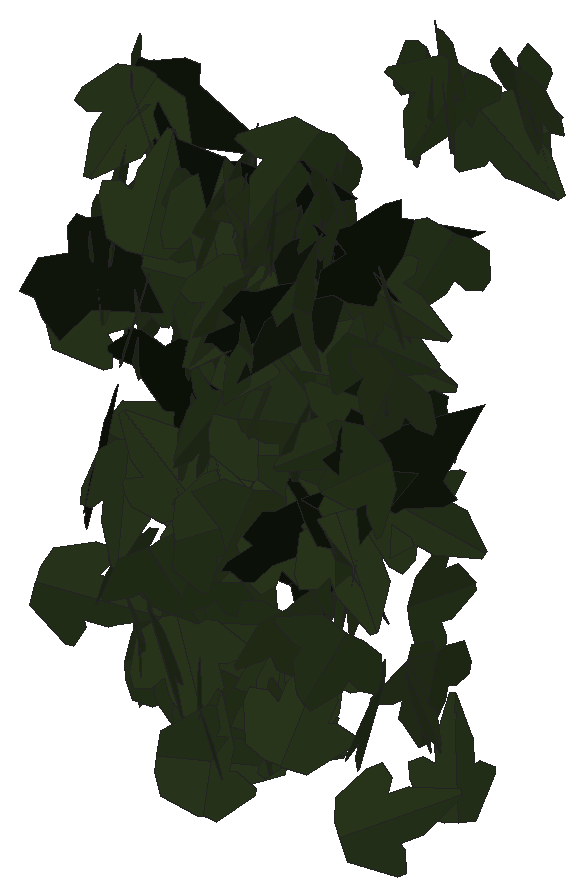
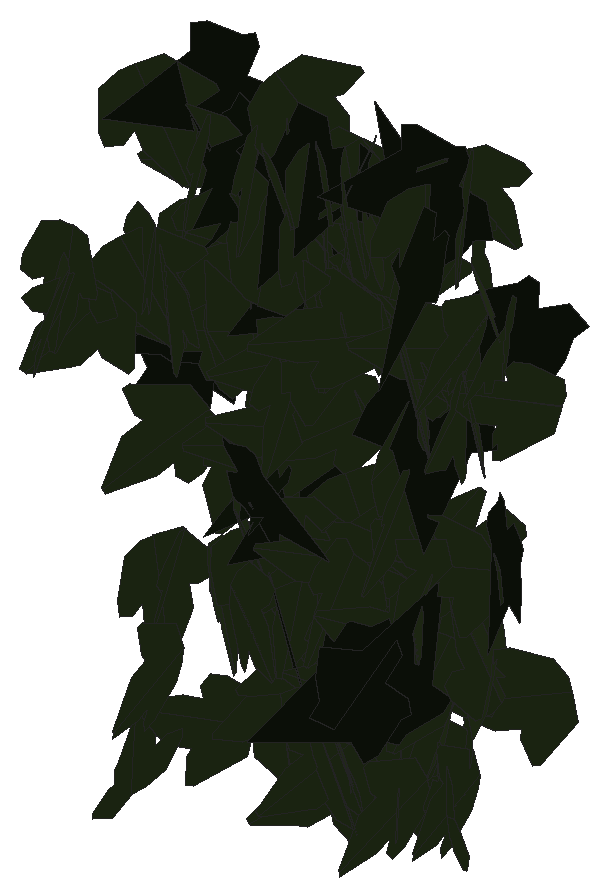
# SketchUp Ruby script. Lengths in inches.
U = 1.inch
M = Sketchup.active_model
def pt(a) = Geom::Point3d.new(a.map { |v| v * U })
def face(e, loops, mat)
  f = e.add_face(loops[0].map { |a| pt(a) })
  loops[1..].each { |l| e.add_face(l.map { |a| pt(a) }).erase! }
  f.material = f.back_material = mat if mat
  f
end
# faces: each face lists its corners as indices into pts; further lists are holes
def faces(e, pts, list, mat = nil) = list.each { |f| face(e, (f[0].is_a?(Array) ? f : [f]).map { |l| l.map { |i| pts[i] } }, mat) }
# xy, xz, yz: faces in a plane at the given z, y or x. An outline is a flat list of corners, or four numbers for a rectangle; further outlines are holes
def ring(l) = l.size == 4 ? [[l[0], l[1]], [l[2], l[1]], [l[2], l[3]], [l[0], l[3]]] : l.each_slice(2).to_a
def flat(e, list, mat, &to3) = list.each { |f| face(e, (f[0].is_a?(Array) ? f : [f]).map { |l| ring(l).map { |u, v| to3.(u, v) } }, mat) }
def xy(e, z, list, mat = nil) = flat(e, list, mat) { |x, y| [x, y, z] }
def xz(e, y, list, mat = nil) = flat(e, list, mat) { |x, z| [x, y, z] }
def yz(e, x, list, mat = nil) = flat(e, list, mat) { |y, z| [x, y, z] }
def lines(e, pts, list) = list.each { |a, b| e.add_line(pt(pts[a]), pt(pts[b])) }
# prism: a flat outline (further loops are holes) pulled along v
def prism(e, loops, v, mat = nil)
  f = face(e, loops, mat); d = Geom::Vector3d.new(v.map { |x| x * U })
  f.pushpull(f.normal.samedirection?(d) ? d.length : -d.length)
end
def box(e, o, s, mat = nil) = prism(e, [[o, [o[0] + s[0], o[1], o[2]], [o[0] + s[0], o[1] + s[1], o[2]], [o[0], o[1] + s[1], o[2]]]], [0, 0, s[2]], mat)
def at(x, y, z, deg = 0) = Geom::Transformation.translation(pt([x, y, z])) * Geom::Transformation.rotation(ORIGIN, Z_AXIS, deg.degrees)
def axes(o, x, y, z) = Geom::Transformation.new([*x, 0, *y, 0, *z, 0, *pt(o).to_a, 1])
def part(name) = M.definitions.add(name)
# library, detail: a bought-in or finely detailed component or shape, given as its bounding box
def library(name, o, s) = part(name).tap { |d| box(d.entities, o, s) }
def detail(e, o, s) = box(e.add_group.entities, o, s)
def put(e, d, t, mat = nil) = e.add_instance(d, t).tap { |i| i.material = mat if mat }
def group(e, t, mat = nil) = e.add_group.tap { |g| g.transformation = t; g.material = mat if mat }.entities
root = M.entities
M.materials.add("efeu1").color = [18, 25, 13]
M.materials.add("efeu2").color = [43, 57, 29]
c1 = part("ivyleaf_9")
p = [[1.54,2.16,1.25],[1.36,2.04,1.19],[-0.21,0.99,0.68],[-0.71,1.11,0.82],[-0.85,0.86,0.67],[-0.8,0.17,0.21],
  [-0.9,-0.01,0.1],[-0.67,-0.16,-0.02],[-0.08,-0.08,-0.05],[-0.03,-0.6,-0.4],[0.65,-0.88,-0.66],[0.83,-0.6,-0.49],
  [1.29,-0.42,-0.43],[1.8125,-0.07,-0.26],[1.21,0.44,0.15]]
faces(c1.entities,p,[[0,1,2,3,4,5,6,7,8,9,10,11,12,13,14]],"efeu1")
c2 = part("ivyleaf_10")
p = [[0,0.5,-0.03],[-0.0625,2.02,-0.43],[-0.19,2.01,-0.46],[-0.54,1.05,-0.29],[-0.52,0.625,-0.18],[-0.83,0.76,-0.28],
  [-1.16,0.64,-0.33],[-1.15,0.33,-0.24],[-0.77,-0.39,0.02],[-0.3,-0.51,0.16],[0.04,-0.48,0.23],[-0.02,2.01,-0.4375],
  [-0.06,2.01,-0.43],[0.04,-0.49,0.23],[0.67,-0.49,0.14],[1.38,0.36,-0.2],[1.375,0.51,-0.24],[0.81,0.65,-0.19],
  [0.62,0.59,-0.15],[0.6,1.09,-0.28],[0.5,1.23,-0.31]]
faces(c2.entities,p,[[0,1,2,3,4,5,6,7,8,9,10],[11,12,0,13,14,15,16,17,18,19,20]],"efeu2")
put(root,c1,axes([22.51,224.58,212.38],[0.06271,-0.08409,-0.48887],[-0.01576,0.49218,-0.08668],[0.4958,0.02628,0.05908]))
put(root,c2,axes([23.38,224.66,212.97],[0.22592,0.39135,-0.21402],[0.09036,0.19477,0.45155],[0.4368,-0.24271,0.01728]))
put(root,c2,axes([26.13,224.89,208.42],[0.18941,-0.45118,-0.10279],[-0.04536,0.09243,-0.48929],[0.46051,0.19467,-0.00592]))
put(root,c2,axes([24.34,225.04,212.48],[0.30249,0.28815,-0.27471],[-0.21033,-0.17727,-0.41754],[-0.33802,0.36817,0.01397]))
put(root,c2,axes([25.64,224.95,208.82],[-0.40532,-0.15765,0.24671],[-0.22122,-0.11108,-0.43442],[0.19178,-0.46131,0.02029]))
put(root,c2,axes([26.13,224.84,211.12],[0.30736,-0.11212,-0.3781],[-0.33453,0.17974,-0.32524],[0.20885,0.4529,0.03547]))
put(root,c2,axes([25.46,224.61,212.77],[-0.1703,0.22314,0.41377],[-0.25775,0.32372,-0.28067],[-0.39314,-0.30889,0.00477]))
put(root,c2,axes([26.38,224.9,212.14],[-0.43486,-0.04069,0.24339],[-0.24112,-0.03479,-0.43663],[0.05247,-0.49713,0.01064]))
put(root,c2,axes([25.77,225.1,211.27],[-0.2106,-0.12766,0.43514],[-0.34341,-0.26845,-0.24496],[0.29618,-0.40204,0.02539]))
put(root,c2,axes([22.2,224.8,208.38],[-0.12391,-0.03449,-0.48317],[0.47025,0.11113,-0.12853],[0.11625,-0.48627,0.0049]))
put(root,c1,axes([26.12,224.55,213.6875],[0.03425,0.24336,-0.43544],[-0.01395,0.43676,0.243],[0.49863,-0.00449,0.0367]))
put(root,c2,axes([24.27,225.04,212.37],[0.07229,-0.49389,0.02911],[0.00313,-0.02896,-0.49915],[0.49474,0.07235,-0.0011]))
put(root,c2,axes([22.88,225,209.91],[0.18698,0.45081,-0.10866],[-0.03926,-0.10135,-0.48804],[-0.46206,0.19104,-0.0025]))
put(root,c2,axes([24.51,224.74,211.96],[0.038,-0.05493,-0.49552],[-0.35423,0.34672,-0.0656],[0.35082,0.35604,-0.01257]))
put(root,c2,axes([25.12,224.77,207.64],[0.29397,0.32785,-0.23685],[0.16042,0.17427,0.44034],[0.37128,-0.33488,-0.00272]))
put(root,c1,axes([25.3,225.11,212.84],[-0.48907,0.07078,-0.07613],[0.07511,-0.01256,-0.49417],[-0.07186,-0.49481,0.00165]))
put(root,c2,axes([23.9375,225.2,213.18],[0.17877,-0.41132,0.22104],[0.10171,-0.1967,-0.44829],[0.45574,0.20524,0.01334]))
put(root,c2,axes([25.97,224.99,213.1],[-0.18972,-0.01175,-0.46246],[0.45973,-0.0605,-0.18706],[-0.05156,-0.49619,0.03376]))
put(root,c2,axes([23.85,224.96,206.61],[0.4903,-0.09038,-0.03797],[0.03745,-0.00629,0.49856],[-0.0906,-0.49172,0.0006]))
put(root,c2,axes([22.71,225.24,208.08],[-0.15403,-0.02039,0.47525],[0.41493,-0.25004,0.12375],[0.23262,0.43251,0.09395]))
put(root,c2,axes([23.98,224.66,209.67],[0.0492,-0.0791,-0.49125],[0.22622,0.44323,-0.04871],[0.44318,-0.21747,0.0794]))
put(root,c2,axes([24.125,224.95,211.59],[0.48591,-0.08464,-0.08204],[0.0858,0.01531,0.49235],[-0.08083,-0.49255,0.02941]))
put(root,c2,axes([24.32,225.1,209.92],[-0.33701,-0.32758,0.17064],[-0.11137,-0.13013,-0.46975],[0.35217,-0.35463,0.01475]))
put(root,c2,axes([24.98,225.23,214.2],[-0.23374,-0.33714,0.28584],[-0.10346,-0.27263,-0.40617],[0.42973,-0.24901,0.05769]))
put(root,c1,axes([23.33,225.2,213.2],[-0.05496,0.02126,0.49651],[0.27897,-0.41209,0.04852],[0.41128,0.28236,0.03344]))
put(root,c2,axes([23.92,224.99,213.36],[0.25014,0.43015,0.04902],[0.02474,0.04232,-0.49759],[-0.43222,0.25136,-0.00011]))
put(root,c2,axes([25.02,225.03,211.14],[-0.13159,0.03096,0.48138],[-0.47888,-0.06829,-0.12652],[0.05791,-0.49435,0.04763]))
put(root,c2,axes([23.77,224.77,206.93],[0.03196,0.02339,0.49843],[0.29196,0.40415,-0.03769],[-0.40464,0.29346,0.01217]))
put(root,c2,axes([22.29,224.82,211.55],[0.13795,-0.00364,-0.48058],[0.41394,0.25493,0.11689],[0.24417,-0.43012,0.07335]))
put(root,c2,axes([23.71,225.1875,212.69],[-0.43376,-0.21923,-0.11744],[-0.09322,-0.07558,0.48538],[-0.23057,0.44298,0.0247]))
put(root,c2,axes([23.63,225.42,210.61],[-0.0463,-0.01692,0.49756],[0.24111,-0.43796,0.00755],[0.43557,0.24063,0.04872]))
put(root,c1,axes([24.55,224.72,212.27],[0.31579,0.25777,0.28954],[0.22934,0.17686,-0.40759],[-0.31254,0.39023,-0.00653]))
put(root,c2,axes([22.5625,225.3125,213.11],[0.25774,-0.26249,0.33862],[0.24668,-0.23218,-0.36775],[0.35031,0.35664,0.00982]))
put(root,c2,axes([23.3125,224.94,209.01],[-0.31521,-0.32538,-0.21159],[0.13739,0.16139,-0.45286],[0.36299,-0.34363,-0.01234]))
put(root,c2,axes([24.6,225.23,213.54],[-0.11233,-0.47313,0.1163],[-0.02337,-0.11399,-0.48627],[0.48666,-0.11468,0.00349]))
put(root,c2,axes([22.89,225.22,214.06],[0.38931,0.20756,-0.23529],[-0.21217,-0.10207,-0.4411],[-0.23114,0.44328,0.0086]))
put(root,c2,axes([24.34,225,212.17],[-0.15774,-0.42128,-0.21827],[0.10073,0.19504,-0.44924],[0.46365,-0.1857,0.02333]))
put(root,c2,axes([25.46,224.96,213.71],[0.26319,-0.24735,-0.34576],[-0.1845,0.2999,-0.35499],[0.383,0.31445,0.06659]))
put(root,c2,axes([24.95,225.03,208.85],[-0.18368,-0.43148,-0.17345],[0.06591,0.16045,-0.46895],[0.46035,-0.19513,-0.00207]))
put(root,c1,axes([24.75,224.74,209.78],[0.23026,0.31315,0.31451],[0.19449,0.24728,-0.38862],[-0.39894,0.30131,-0.00793]))
put(root,c2,axes([25.03,225.27,209.52],[-0.18872,0.04853,0.46046],[0.44596,-0.11467,0.19486],[0.12452,0.48425,0]))
put(root,c2,axes([22.39,225.25,212.4375],[-0.08525,0.43997,-0.22172],[0.04727,-0.21668,-0.44813],[-0.49041,-0.09737,-0.00465]))
put(root,c2,axes([22.89,225.16,211.84],[0.27516,-0.40484,-0.10194],[-0.05052,0.08891,-0.48943],[0.41441,0.27965,0.00802]))
put(root,c2,axes([25.08,225.25,211.25],[0.16639,-0.47051,0.03052],[0.01197,-0.02814,-0.49906],[0.47135,0.16681,0.0019]))
put(root,c2,axes([22.63,225.14,208.53],[0.13985,-0.4761,0.06142],[0.01597,0.06855,0.49502],[-0.47978,-0.1365,0.03438]))
put(root,c1,axes([22.62,224.86,210.01],[-0.06368,0.06353,-0.49184],[-0.42731,0.24464,0.08692],[0.25169,0.43141,0.02314]))
put(root,c2,axes([23.88,224.97,207.41],[-0.29424,0.24931,0.31822],[-0.27089,0.17056,-0.3841],[-0.30007,-0.39844,0.0347]))
put(root,c2,axes([26.74,225.27,213.65],[-0.36974,-0.24254,0.23337],[-0.18399,-0.14464,-0.44184],[0.28184,-0.41261,0.01771]))
put(root,c2,axes([25.53,225.12,209.95],[0.38768,0.24698,0.19674],[0.16239,0.11123,-0.45963],[-0.2708,0.42027,0.00603]))
put(root,c2,axes([23.2,225.1,208.11],[-0.36099,0.34569,0.01376],[-0.01056,0.00886,-0.49981],[-0.3458,-0.36114,0.00091]))
put(root,c1,axes([25.58,225.05,213.31],[0.4787,-0.00945,-0.14406],[-0.14405,0.00219,-0.4788],[0.00968,0.49991,-0.00062]))
put(root,c2,axes([23.34,225.31,209.6875],[0.26007,0.33545,0.26427],[-0.15962,-0.21063,0.42445],[0.39609,-0.30513,-0.00247]))
put(root,c1,axes([23.3,225.09,211.35],[0.33474,0.27089,-0.25409],[-0.20615,-0.14903,-0.43046],[-0.30895,0.39295,0.01192]))
put(root,c2,axes([24.5625,225.25,213.54],[0.30258,-0.39488,-0.05015],[0.03957,0.09253,-0.48977],[0.39608,0.29242,0.08724]))
put(root,c2,axes([26.21,225.04,213.18],[-0.25662,0.35379,0.24286],[-0.15972,0.1839,-0.43666],[-0.39829,-0.30169,0.01863]))
put(root,c2,axes([25.91,224.99,206.84],[0.09338,0.07372,-0.48564],[0.39843,0.27775,0.11877],[0.28729,-0.40917,-0.00687]))
put(root,c2,axes([24.09,225.22,209.21],[0.43803,0.21189,0.11504],[-0.10595,-0.04514,0.48656],[0.21658,-0.45063,0.00536]))
put(root,c1,axes([25.02,225.28,210.16],[0.38205,-0.32072,-0.03431],[-0.02242,0.02665,-0.49879],[0.32177,0.38266,0.00598]))
put(root,c2,axes([25.14,225.04,212.22],[-0.11647,-0.12041,0.4711],[0.3004,0.36311,0.16707],[-0.38236,0.32195,-0.01225]))
put(root,c2,axes([24.38,224.93,213.27],[0.0063,0.16368,-0.47241],[-0.13171,0.4563,0.15634],[0.4823,0.12247,0.04887]))
put(root,c1,axes([25.98,225.2,210.76],[-0.07751,-0.07617,0.48805],[0.4934,-0.03535,0.07285],[0.0234,0.4929,0.08064]))
put(root,c2,axes([25.86,225.06,212.41],[-0.18763,-0.25465,-0.38723],[0.2358,0.3072,-0.31627],[0.39899,-0.3013,0.00482]))
put(root,c2,axes([25.81,225.63,211.87],[-0.0072,0.03274,-0.49888],[0.17465,-0.46733,-0.03319],[-0.46845,-0.17473,-0.00471]))
put(root,c2,axes([25.32,225.51,209.5],[0.33907,-0.28409,0.23308],[0.17173,-0.15788,-0.44225],[0.32488,0.37996,-0.00949]))
put(root,c2,axes([24.1,225.55,207.3125],[0.18188,-0.20237,-0.41948],[0.27058,-0.32063,0.272],[-0.37909,-0.32595,-0.00712]))
put(root,c2,axes([24.1,225.35,213.6875],[0.15528,-0.47066,-0.06612],[-0.00867,0.06675,-0.49545],[0.4752,0.15501,0.01257]))
put(root,c2,axes([23.5,225.18,211.49],[0.17279,-0.0674,0.46433],[-0.4374,0.15591,0.1854],[-0.16978,-0.47026,-0.00508]))
put(root,c2,axes([26.48,225.14,208.58],[-0.26061,0.37016,0.21227],[-0.12667,0.17041,-0.45268],[-0.40748,-0.28972,0.00495]))
put(root,c1,axes([25.96,225.57,211.4375],[-0.33858,-0.35305,-0.10354],[0.07191,0.0745,-0.48916],[0.36082,-0.34613,0.00033]))
put(root,c2,axes([24.25,225.06,210.86],[0.11549,0.10713,0.47454],[0.20491,0.43164,-0.14732],[-0.44122,0.2285,0.0558]))
put(root,c2,axes([23.125,225.28,208.64],[-0.40969,-0.22091,-0.18264],[0.16015,0.0878,-0.46545],[0.23771,-0.43988,-0.00118]))
put(root,c2,axes([22.98,225.27,212.12],[-0.08588,-0.0268,-0.49184],[0.48576,0.07811,-0.08907],[0.08161,-0.49313,0.01262]))
put(root,c2,axes([25.7,225.25,212.55],[0.29909,-0.22386,-0.33231],[-0.21001,0.26558,-0.36792],[0.34124,0.35966,0.06483]))
put(root,c2,axes([25.05,225.24,210.33],[0.07468,0.0104,0.49428],[0.41447,0.27119,-0.06833],[-0.26951,0.41994,0.03188]))
put(root,c2,axes([26.43,225.44,208.64],[-0.12758,-0.4834,0.00685],[-0.00053,-0.00694,-0.49995],[0.48345,-0.12757,0.00126]))
put(root,c2,axes([23.26,225.36,207.88],[0.41284,0.22808,0.16595],[0.14003,0.08963,-0.47155],[-0.24485,0.43583,0.01013]))
put(root,c2,axes([24.7,225.24,210.6],[-0.00821,-0.00816,-0.49987],[0.47653,0.15104,-0.01029],[0.15116,-0.47657,0.00529]))
put(root,c2,axes([22.57,225.42,209.91],[-0.12024,0.00671,-0.48528],[0.48113,-0.06394,-0.1201],[-0.06367,-0.49585,0.00892]))
put(root,c1,axes([24.51,225.24,213.72],[0.43005,0.24075,-0.08426],[-0.0724,-0.04317,-0.49284],[-0.24458,0.43609,-0.00227]))
put(root,c2,axes([24.95,225.53,213.51],[0.3428,-0.36365,-0.01576],[-0.00089,0.0208,-0.49957],[0.36399,0.34253,0.01361]))
put(root,c2,axes([24.55,225.54,213.03],[0.01697,-0.49932,0.01977],[0.01918,-0.01912,-0.49927],[0.49934,0.0177,0.01851]))
put(root,c2,axes([22.8,225.3125,209.77],[0.26349,0.27008,0.32807],[0.23811,0.22589,-0.37719],[-0.35196,0.35501,-0.00958]))
put(root,c2,axes([23.08,225.53,213.71],[-0.28342,-0.41191,0.00025],[0.07557,-0.05229,-0.49148],[0.40492,-0.27855,0.0919]))
put(root,c2,axes([24.19,225.43,207.02],[0.46244,-0.18954,-0.01487],[0.02278,0.01639,0.49921],[-0.18876,-0.46239,0.0238]))
put(root,c1,axes([22.86,225.375,214],[0.12553,0.0359,-0.48265],[0.33172,0.3567,0.11281],[0.35243,-0.34853,0.06573]))
put(root,c2,axes([22.79,225.28,214.03],[-0.25972,0.25553,0.34242],[-0.26486,0.21814,-0.36368],[-0.33525,-0.37029,0.02205]))
put(root,c2,axes([24.53,225.33,209.6],[0.25206,0.25044,0.35177],[0.22433,0.2721,-0.35446],[-0.36898,0.33651,0.02481]))
put(root,c2,axes([23.26,225.57,212.01],[0.27885,-0.40427,-0.09387],[-0.05636,0.07516,-0.49109],[0.41118,0.28446,-0.00366]))
put(root,c2,axes([25.41,225.55,212.25],[-0.35665,-0.3484,-0.03768],[0.02213,0.03126,-0.49853],[0.34973,-0.35727,-0.00688]))
put(root,c2,axes([24.69,225.44,211.3],[-0.14813,-0.42064,-0.22611],[0.09545,0.20588,-0.44554],[0.46792,-0.17516,0.01931]))
put(root,c2,axes([23.86,225.44,208.9],[-0.27105,-0.35416,-0.22606],[0.13274,0.18306,-0.44595],[0.39864,-0.30176,-0.00522]))
put(root,c2,axes([22.88,225.22,211.47],[0.02949,-0.07999,-0.49268],[-0.05445,0.49008,-0.08282],[0.49615,0.05854,0.02019]))
put(root,c2,axes([25.11,225.51,213.65],[0.04827,-0.46156,-0.18609],[0.08218,0.19179,-0.45438],[0.49083,0.01329,0.09438]))
put(root,c1,axes([25.04,225.4,208.72],[-0.14925,0.05487,-0.47404],[-0.46587,0.09083,0.1572],[0.10336,0.48861,0.02401]))
put(root,c2,axes([22.51,225.82,207.39],[0.18153,-0.07651,0.45956],[0.42907,-0.16471,-0.19691],[0.18152,0.46585,0.00585]))
put(root,c2,axes([23.375,225.34,209.21],[0.07792,0.00103,-0.49389],[-0.242,0.43594,-0.03727],[0.43054,0.24485,0.06843]))
put(root,c2,axes([24.89,225.73,212.43],[-0.49926,0.00064,-0.02727],[-0.02728,-0.01362,0.49907],[-0.0001,0.49981,0.01363]))
put(root,c2,axes([23.96,225.4375,209.49],[0.13425,-0.02686,-0.48089],[0.42634,0.23888,0.10569],[0.22407,-0.43842,0.08704]))
put(root,c2,axes([23.6,225.52,208.09],[-0.08789,-0.05538,0.48909],[0.41449,0.25963,0.10389],[-0.26547,0.4237,0.00027]))
put(root,c2,axes([24.49,225.52,211.61],[-0.11943,-0.09905,-0.47532],[0.45415,0.15031,-0.14543],[0.1717,-0.46647,0.05407]))
put(root,c2,axes([24.14,225.44,207.13],[-0.16299,-0.15367,-0.44701],[0.34708,0.28208,-0.22352],[0.32089,-0.38317,0.01472]))
put(root,c2,axes([23.38,225.42,208.84],[0.13135,0.15005,-0.45851],[0.33561,0.31296,0.19856],[0.34658,-0.35992,-0.0185]))
put(root,c2,axes([26.06,225.46,210.3],[0.1921,0.20276,0.41471],[0.15775,0.39331,-0.26537],[-0.43383,0.2328,0.08714]))
put(root,c2,axes([24.01,225.46,212],[0.02334,-0.03811,0.498],[0.24085,0.43761,0.0222],[-0.43755,0.23885,0.03878]))
put(root,c2,axes([22.65,225.4,212.46],[-0.0705,0.16971,0.465],[-0.16105,0.43627,-0.18365],[-0.46807,-0.17567,-0.00685]))
put(root,c2,axes([23.3125,225.55,210.47],[0.08962,-0.33726,-0.35809],[0.06496,0.36891,-0.33119],[0.48759,0.01284,0.10994]))
put(root,c2,axes([24.04,225.57,207.47],[-0.18282,-0.21343,-0.41355],[0.2945,0.29098,-0.28036],[0.36035,-0.34609,0.01932]))
put(root,c2,axes([23.9375,225.61,209.5],[-0.07608,-0.36285,-0.33548],[0.07778,0.32641,-0.37068],[0.48802,-0.10859,0.00678]))
put(root,c2,axes([22.6875,225.46,207.44],[-0.01189,0.07995,0.49342],[-0.19878,0.4521,-0.07805],[-0.45864,-0.19802,0.02104]))
put(root,c2,axes([24.54,225.89,207.88],[0.32909,0.37318,-0.04933],[-0.0355,-0.03446,-0.49755],[-0.37475,0.33098,0.00381]))
put(root,c2,axes([23.33,225.51,207.17],[0.01391,0.19707,0.45931],[-0.07049,0.45567,-0.19337],[-0.49481,-0.05937,0.04046]))
put(root,c2,axes([25.29,225.76,211.73],[0.07338,-0.01197,0.49444],[0.43784,0.23405,-0.05931],[-0.23003,0.44168,0.04482]))
put(root,c2,axes([23.8,225.93,207.08],[0.42511,-0.2473,-0.09012],[0.08238,-0.03759,0.49173],[-0.24999,-0.43293,0.00878]))
put(root,c1,axes([23.25,226.1,208.41],[0.21561,0.13787,0.42954],[-0.40558,-0.14922,0.25148],[0.19753,-0.45687,0.04749]))
put(root,c1,axes([25.07,225.85,210.24],[-0.1973,-0.03723,-0.45791],[-0.45169,-0.07533,0.20075],[-0.08394,0.49289,-0.00391]))
put(root,c1,axes([22.6875,225.95,213.64],[0.37881,-0.07131,-0.31846],[-0.30562,0.09361,-0.3845],[0.11446,0.48596,0.02733]))
put(root,c2,axes([24.93,225.99,208.96],[0.16988,-0.06007,-0.46641],[-0.31485,0.35382,-0.16024],[0.3493,0.34814,0.08239]))
put(root,c1,axes([23.18,226.11,208.73],[0.46642,0.00645,0.18002],[0.18002,0.00146,-0.46647],[-0.00654,0.49996,-0.00096]))
put(root,c2,axes([26.07,226.23,206.7],[0.05047,0.46617,-0.17362],[-0.0201,0.17628,0.46746],[0.49704,-0.04021,0.03653]))
put(root,c2,axes([25.34,226.7,208.4375],[-0.02271,0.10809,0.48765],[-0.17903,0.45396,-0.10896],[-0.4663,-0.17956,0.01808]))
put(root,c2,axes([24.75,227.95,213.64],[-0.32179,-0.28522,0.25515],[-0.1649,-0.19748,-0.42873],[0.34534,-0.36007,0.03303]))
put(root,c2,axes([24.54,227.99,213.93],[-0.36127,0.32098,-0.1283],[0.03244,-0.15328,-0.47482],[-0.34414,-0.3514,0.08992]))
put(root,c2,axes([24.21,228.01,213.59],[0.40783,-0.28139,0.06703],[0.099,0.02691,-0.48936],[0.27179,0.41243,0.07766]))
put(root,c2,axes([24.99,228.25,213.17],[-0.35199,-0.17532,-0.30881],[0.32036,0.0308,-0.38265],[0.1532,-0.46724,0.09065]))
put(root,c2,axes([25.3,228.29,213.71],[-0.47171,0.15217,0.06587],[-0.06779,0.0043,-0.49536],[-0.15132,-0.47626,0.01658]))
put(root,c2,axes([25.1,228.66,213.51],[-0.24716,0.4342,-0.0197],[0.01614,-0.01348,-0.49956],[-0.43434,-0.24757,-0.00735]))
